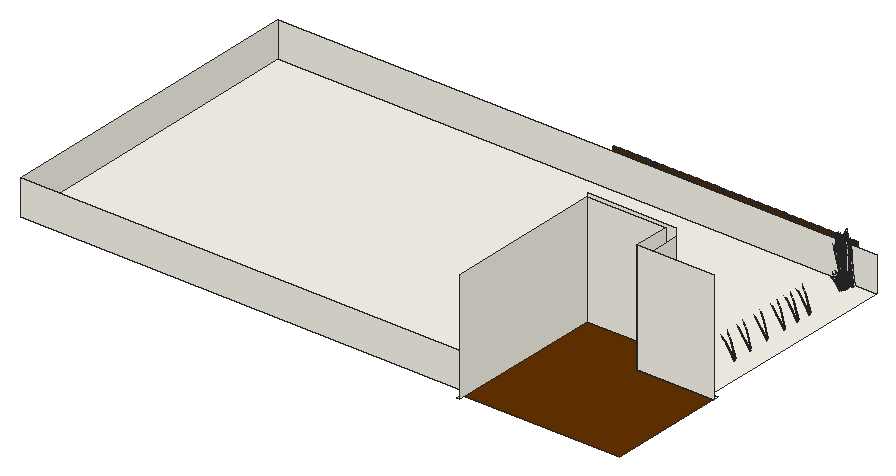
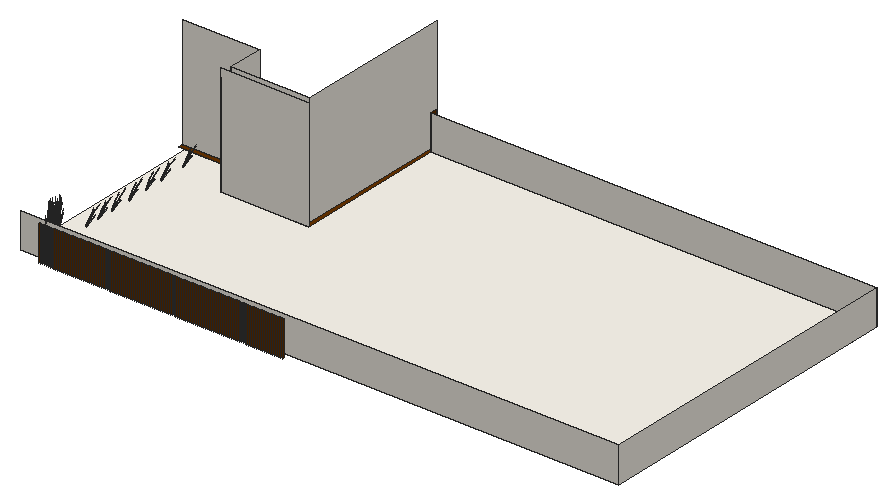
# SketchUp Ruby script. Lengths in inches.
U = 1.inch
M = Sketchup.active_model
def pt(a) = Geom::Point3d.new(a.map { |v| v * U })
def face(e, loops, mat)
  f = e.add_face(loops[0].map { |a| pt(a) })
  loops[1..].each { |l| e.add_face(l.map { |a| pt(a) }).erase! }
  f.material = f.back_material = mat if mat
  f
end
# faces: each face lists its corners as indices into pts; further lists are holes
def faces(e, pts, list, mat = nil) = list.each { |f| face(e, (f[0].is_a?(Array) ? f : [f]).map { |l| l.map { |i| pts[i] } }, mat) }
# xy, xz, yz: faces in a plane at the given z, y or x. An outline is a flat list of corners, or four numbers for a rectangle; further outlines are holes
def ring(l) = l.size == 4 ? [[l[0], l[1]], [l[2], l[1]], [l[2], l[3]], [l[0], l[3]]] : l.each_slice(2).to_a
def flat(e, list, mat, &to3) = list.each { |f| face(e, (f[0].is_a?(Array) ? f : [f]).map { |l| ring(l).map { |u, v| to3.(u, v) } }, mat) }
def xy(e, z, list, mat = nil) = flat(e, list, mat) { |x, y| [x, y, z] }
def xz(e, y, list, mat = nil) = flat(e, list, mat) { |x, z| [x, y, z] }
def yz(e, x, list, mat = nil) = flat(e, list, mat) { |y, z| [x, y, z] }
def lines(e, pts, list) = list.each { |a, b| e.add_line(pt(pts[a]), pt(pts[b])) }
# prism: a flat outline (further loops are holes) pulled along v
def prism(e, loops, v, mat = nil)
  f = face(e, loops, mat); d = Geom::Vector3d.new(v.map { |x| x * U })
  f.pushpull(f.normal.samedirection?(d) ? d.length : -d.length)
end
def box(e, o, s, mat = nil) = prism(e, [[o, [o[0] + s[0], o[1], o[2]], [o[0] + s[0], o[1] + s[1], o[2]], [o[0], o[1] + s[1], o[2]]]], [0, 0, s[2]], mat)
def at(x, y, z, deg = 0) = Geom::Transformation.translation(pt([x, y, z])) * Geom::Transformation.rotation(ORIGIN, Z_AXIS, deg.degrees)
def axes(o, x, y, z) = Geom::Transformation.new([*x, 0, *y, 0, *z, 0, *pt(o).to_a, 1])
def part(name) = M.definitions.add(name)
# library, detail: a bought-in or finely detailed component or shape, given as its bounding box
def library(name, o, s) = part(name).tap { |d| box(d.entities, o, s) }
def detail(e, o, s) = box(e.add_group.entities, o, s)
def put(e, d, t, mat = nil) = e.add_instance(d, t).tap { |i| i.material = mat if mat }
def group(e, t, mat = nil) = e.add_group.tap { |g| g.transformation = t; g.material = mat if mat }.entities
root = M.entities
M.materials.add("C01_Vanilla_Cream").color = [255, 251, 241]
M.materials.add("C08_Toffee_Ember").color = [102, 51, 0]
M.materials.add("LightPink_Translucent").color = [144, 107, 117]
M.materials["LightPink_Translucent"].alpha = 0.75
c1 = part("blade")
p = [[2.15,0.21,22],[0,0.17,0],[0.09,0.45,0],[2.18,0.31,22],[2.29,0.31,22],[0.38,0.45,0],
  [2.48,0.24,33],[2.49,0.24,33],[2.48,0.22,33]]
faces(c1.entities,p,[[0,1,2,3],[4,5,2,3],[6,3,4,7],[8,0,3,6]])
c2 = part("seeds")
p = [[0.3,-0.1,1.38],[-0.01,-0.03,1.59],[-0.01,-0.03,0.03],[0.14,-0.07,-0.07],[0.29,-0.03,3],[0.15,0.01,3.11]]
faces(c2.entities,p,[[0,1,2,3],[1,0,4,5]],"LightPink_Translucent")
c3 = part("blade with seeds")
put(c3.entities,c1,at(0,0,0))
put(c3.entities,c2,axes([2.4,0.25,30.99],[1.5799,-0.05474,1.17369],[-0.12525,1.92788,0.29478],[-0.07173,-0.02425,1.56792]))
xy(root,510,[[531,12,531,180,621.41,180,621.41,144,693.41,144,693.41,138,615.41,138,615.41,174,535,174,535,12],[75,24,531,24,531,180,621.41,180,621.41,144,687.41,144,687.41,354,75,354]],"C01_Vanilla_Cream")
xy(root,510,[[531,18,693.41,18,693.41,144,621.41,144,621.41,180,531,180]],"C08_Toffee_Ember")
xz(root,24,[[75,510,531,546]],"C01_Vanilla_Cream")
xz(root,138,[[615.41,510,693.41,624]],"C01_Vanilla_Cream")
xz(root,174,[[535,510,615.41,624]],"C01_Vanilla_Cream")
xz(root,180,[[531,510,621.41,624]],"C01_Vanilla_Cream")
xz(root,354,[[75,510,687.41,546]],"C01_Vanilla_Cream")
yz(root,75,[[24,510,354,546]],"C01_Vanilla_Cream")
yz(root,413.02,[[360,510,361.11,546]],"C08_Toffee_Ember")
yz(root,415.03,[[360,510,361.11,546]],"C08_Toffee_Ember")
yz(root,417.05,[[360,510,361.11,546]],"C08_Toffee_Ember")
yz(root,419.07,[[360,510,361.11,546]],"C08_Toffee_Ember")
yz(root,421.09,[[360,510,361.11,546]],"C08_Toffee_Ember")
yz(root,423.1,[[360,510,361.11,546]],"C08_Toffee_Ember")
yz(root,425.12,[[360,510,361.11,546]],"C08_Toffee_Ember")
yz(root,427.14,[[360,510,361.11,546]],"C08_Toffee_Ember")
yz(root,429.16,[[360,510,361.09,546]],"C08_Toffee_Ember")
yz(root,431.17,[[360,510,361.09,546]],"C08_Toffee_Ember")
yz(root,433.19,[[360,510,361.09,546]],"C08_Toffee_Ember")
yz(root,435.21,[[360,510,361.09,546]],"C08_Toffee_Ember")
yz(root,437.22,[[360,510,361.09,546]],"C08_Toffee_Ember")
yz(root,439.24,[[360,510,361.09,546]],"C08_Toffee_Ember")
yz(root,441.26,[[360,510,361.09,546]],"C08_Toffee_Ember")
yz(root,443.28,[[360,510,361.09,546]],"C08_Toffee_Ember")
yz(root,445.29,[[360,510,361.09,546]],"C08_Toffee_Ember")
yz(root,447.31,[[360,510,361.09,546]],"C08_Toffee_Ember")
yz(root,449.33,[[360,510,361.09,546]],"C08_Toffee_Ember")
yz(root,451.34,[[360,510,361.09,546]],"C08_Toffee_Ember")
yz(root,453.36,[[360,510,361.09,546]],"C08_Toffee_Ember")
yz(root,455.38,[[360,510,361.09,546]],"C08_Toffee_Ember")
yz(root,457.4,[[360,510,361.09,546]],"C08_Toffee_Ember")
yz(root,459.41,[[360,510,361.09,546]],"C08_Toffee_Ember")
yz(root,461.43,[[360,510,361.09,546]],"C08_Toffee_Ember")
yz(root,463.45,[[360,510,361.09,546]],"C08_Toffee_Ember")
yz(root,465.47,[[360,510,361.09,546]],"C08_Toffee_Ember")
yz(root,467.48,[[360,510,361.09,546]],"C08_Toffee_Ember")
yz(root,469.5,[[360,510,361.09,546]],"C08_Toffee_Ember")
yz(root,471.52,[[360,510,361.09,546]],"C08_Toffee_Ember")
yz(root,473.53,[[360,510,361.1875,546]],"C08_Toffee_Ember")
yz(root,475.55,[[360,510,361.1875,546]],"C08_Toffee_Ember")
yz(root,477.57,[[360,510,361.1875,546]],"C08_Toffee_Ember")
yz(root,479.59,[[360,510,361.1875,546]],"C08_Toffee_Ember")
yz(root,481.6,[[360,510,361.1875,546]],"C08_Toffee_Ember")
yz(root,483.62,[[360,510,361.1875,546]],"C08_Toffee_Ember")
yz(root,485.64,[[360,510,361.1875,546]],"C08_Toffee_Ember")
yz(root,487.66,[[360,510,361.1875,546]],"C08_Toffee_Ember")
yz(root,489.67,[[360,510,361.1875,546]],"C08_Toffee_Ember")
yz(root,491.69,[[360,510,361.1875,546]],"C08_Toffee_Ember")
yz(root,493.71,[[360,510,361.1875,546]],"C08_Toffee_Ember")
yz(root,495.72,[[360,510,361.1875,546]],"C08_Toffee_Ember")
yz(root,497.74,[[360,510,361.1875,546]],"C08_Toffee_Ember")
yz(root,499.76,[[360,510,361.1875,546]],"C08_Toffee_Ember")
yz(root,501.78,[[360,510,361.1875,546]],"C08_Toffee_Ember")
yz(root,503.79,[[360,510,361.1875,546]],"C08_Toffee_Ember")
yz(root,505.81,[[360,510,361.1875,546]],"C08_Toffee_Ember")
yz(root,507.83,[[360,510,361.1875,546]],"C08_Toffee_Ember")
yz(root,509.84,[[360,510,361.1875,546]],"C08_Toffee_Ember")
yz(root,511.86,[[360,510,361.1875,546]],"C08_Toffee_Ember")
yz(root,513.88,[[360,510,361.1875,546]],"C08_Toffee_Ember")
yz(root,515.9,[[360,510,361.1875,546]],"C08_Toffee_Ember")
yz(root,517.91,[[360,510,361.1875,546]],"C08_Toffee_Ember")
yz(root,519.93,[[360,510,361.1875,546]],"C08_Toffee_Ember")
yz(root,521.95,[[360,510,361.1875,546]],"C08_Toffee_Ember")
yz(root,523.97,[[360,510,361.1875,546]],"C08_Toffee_Ember")
yz(root,525.98,[[360,510,361.1875,546]],"C08_Toffee_Ember")
yz(root,528,[[360,510,361.1875,546]],"C08_Toffee_Ember")
yz(root,530.02,[[360,510,361.1875,546]],"C08_Toffee_Ember")
yz(root,531,[[18,510,24,546]],"C08_Toffee_Ember")
yz(root,532.03,[[360,510,361.1875,546]],"C08_Toffee_Ember")
yz(root,534.05,[[360,510,361.1875,546]],"C08_Toffee_Ember")
yz(root,535,[[12,510,174,624]],"C01_Vanilla_Cream")
yz(root,536.07,[[360,510,361.1875,546]],"C08_Toffee_Ember")
yz(root,538.09,[[360,510,361.1875,546]],"C08_Toffee_Ember")
yz(root,540.1,[[360,510,361.1875,546]],"C08_Toffee_Ember")
yz(root,542.12,[[360,510,361.1875,546]],"C08_Toffee_Ember")
yz(root,544.14,[[360,510,361.1875,546]],"C08_Toffee_Ember")
yz(root,546.15,[[360,510,361.1875,546]],"C08_Toffee_Ember")
yz(root,548.17,[[360,510,361.1875,546]],"C08_Toffee_Ember")
yz(root,550.1875,[[360,510,361.1875,546]],"C08_Toffee_Ember")
yz(root,552.21,[[360,510,361.1875,546]],"C08_Toffee_Ember")
yz(root,554.22,[[360,510,361.1875,546]],"C08_Toffee_Ember")
yz(root,556.24,[[360,510,361.1875,546]],"C08_Toffee_Ember")
yz(root,558.26,[[360,510,361.1875,546]],"C08_Toffee_Ember")
yz(root,560.28,[[360,510,361.1875,546]],"C08_Toffee_Ember")
yz(root,562.29,[[360,510,361.1875,546]],"C08_Toffee_Ember")
yz(root,564.31,[[360,510,361.1875,546]],"C08_Toffee_Ember")
yz(root,566.33,[[360,510,361.1875,546]],"C08_Toffee_Ember")
yz(root,568.34,[[360,510,361.1875,546]],"C08_Toffee_Ember")
yz(root,570.36,[[360,510,361.1875,546]],"C08_Toffee_Ember")
yz(root,572.38,[[360,510,361.1875,546]],"C08_Toffee_Ember")
yz(root,574.4,[[360,510,361.1875,546]],"C08_Toffee_Ember")
yz(root,576.41,[[360,510,361.1875,546]],"C08_Toffee_Ember")
yz(root,578.43,[[360,510,361.1875,546]],"C08_Toffee_Ember")
yz(root,580.45,[[360,510,361.1875,546]],"C08_Toffee_Ember")
yz(root,582.47,[[360,510,361.1875,546]],"C08_Toffee_Ember")
yz(root,584.48,[[360,510,361.1875,546]],"C08_Toffee_Ember")
yz(root,586.5,[[360,510,361.1875,546]],"C08_Toffee_Ember")
yz(root,588.52,[[360,510,361.1875,546]],"C08_Toffee_Ember")
yz(root,590.53,[[360,510,361.1875,546]],"C08_Toffee_Ember")
yz(root,592.55,[[360,510,361.1875,546]],"C08_Toffee_Ember")
yz(root,594.57,[[360,510,361.1875,546]],"C08_Toffee_Ember")
yz(root,596.59,[[360,510,361.1875,546]],"C08_Toffee_Ember")
yz(root,598.6,[[360,510,361.13,546]],"C08_Toffee_Ember")
yz(root,600.62,[[360,510,361.13,546]],"C08_Toffee_Ember")
yz(root,602.64,[[360,510,361.13,546]],"C08_Toffee_Ember")
yz(root,604.65,[[360,510,361.13,546]],"C08_Toffee_Ember")
yz(root,606.67,[[360,510,361.13,546]],"C08_Toffee_Ember")
yz(root,608.6875,[[360,510,361.13,546]],"C08_Toffee_Ember")
yz(root,610.71,[[360,510,361.13,546]],"C08_Toffee_Ember")
yz(root,612.72,[[360,510,361.13,546]],"C08_Toffee_Ember")
yz(root,614.74,[[360,510,361.13,546]],"C08_Toffee_Ember")
yz(root,615.41,[[138,510,174,624]],"C01_Vanilla_Cream")
yz(root,616.76,[[360,510,361.13,546]],"C08_Toffee_Ember")
yz(root,618.78,[[360,510,361.13,546]],"C08_Toffee_Ember")
yz(root,620.79,[[360,510,361.13,546]],"C08_Toffee_Ember")
yz(root,621.41,[[144,510,180,615]],"C01_Vanilla_Cream")
yz(root,622.81,[[360,510,361.13,546]],"C08_Toffee_Ember")
yz(root,624.83,[[360,510,361.13,546]],"C08_Toffee_Ember")
yz(root,626.84,[[360,510,361.13,546]],"C08_Toffee_Ember")
yz(root,628.86,[[360,510,361.13,546]],"C08_Toffee_Ember")
yz(root,630.88,[[360,510,361.13,546]],"C08_Toffee_Ember")
yz(root,632.9,[[360,510,361.13,546]],"C08_Toffee_Ember")
yz(root,634.91,[[360,510,361.13,546]],"C08_Toffee_Ember")
yz(root,636.93,[[360,510,361.13,546]],"C08_Toffee_Ember")
yz(root,638.95,[[360,510,361.13,546]],"C08_Toffee_Ember")
yz(root,640.97,[[360,510,361.13,546]],"C08_Toffee_Ember")
yz(root,642.98,[[360,510,361,546]],"C08_Toffee_Ember")
yz(root,645,[[360,510,361,546]],"C08_Toffee_Ember")
yz(root,647.02,[[360,510,361,546]],"C08_Toffee_Ember")
yz(root,649.03,[[360,510,361,546]],"C08_Toffee_Ember")
yz(root,651.05,[[360,510,361,546]],"C08_Toffee_Ember")
yz(root,653.07,[[360,510,361,546]],"C08_Toffee_Ember")
yz(root,655.09,[[360,510,361,546]],"C08_Toffee_Ember")
yz(root,657.1,[[360,510,361,546]],"C08_Toffee_Ember")
yz(root,659.12,[[360,510,361,546]],"C08_Toffee_Ember")
yz(root,661.14,[[360,510,361,546]],"C08_Toffee_Ember")
yz(root,663.15,[[360,510,361,546]],"C08_Toffee_Ember")
put(root,c3,axes([662.41,340.34,511.24],[0.0165,0.08998,1.46364],[-0.33262,0.46992,-0.2236],[-0.23626,-0.02369,0.24931]))
put(root,c3,axes([662.23,342.86,511.24],[0.08727,0.05704,1.46364],[0.14797,0.52853,-0.2236],[-0.19341,0.11271,0.24931]))
put(root,c3,axes([665.12,347.62,512.15],[0.12702,0.15896,1.18691],[-0.2927,0.4321,-0.25526],[-0.30054,-0.10328,0.50747]))
put(root,c3,axes([664.59,341.16,511.71],[-0.67676,-0.09361,-0.51753],[0.14281,-0.57742,-0.13583],[-0.20196,-0.06997,1.14236]))
put(root,c3,axes([664.67,348.68,511.24],[0.0165,0.08998,1.46364],[-0.33262,0.46992,-0.2236],[-0.23626,-0.02369,0.24931]))
put(root,c3,axes([663.7,342.25,511.67],[-0.60889,-0.28548,-0.4121],[0.36394,-0.51192,0],[-0.13868,-0.06502,1.30728]))
put(root,c3,axes([663.43,338,511.24],[-0.06302,0.07522,1.46364],[-0.63686,0.16217,-0.2236],[-0.15385,-0.14752,0.24931]))
put(root,c3,axes([664.07,342.59,511.97],[-0.40676,0.57214,0],[-0.68052,-0.31907,-0.42834],[-0.15499,-0.07267,1.3588]))
put(root,c3,axes([663.03,338.29,511.77],[-0.18768,0.46622,-0.03231],[-0.57763,-0.14342,-0.14649],[-0.0877,-0.07626,0.48318]))
put(root,c3,axes([664.49,351.2,511.24],[0.08727,0.05704,1.46364],[0.14797,0.52853,-0.2236],[-0.19341,0.11271,0.24931]))
put(root,c3,axes([665.35,341.24,512.21],[-0.65687,0.37907,-0.24149],[-0.43681,-0.53562,-0.41502],[-0.16207,-0.0544,1.32557]))
put(root,c3,axes([662.72,340.42,511.97],[-0.81352,0,0],[0,-0.63814,-0.42834],[0,-0.14534,1.3588]))
put(root,c3,axes([663.87,342.04,511.68],[-0.15283,-0.49751,-0.25712],[0.60696,-0.14127,0.25712],[-0.12236,-0.05737,1.15348]))
put(root,c3,axes([665.79,341.66,511.71],[-0.43821,0.42916,-0.51753],[-0.54436,-0.38915,-0.13583],[-0.1756,0.10706,1.14236]))
put(root,c3,axes([663.35,340.25,511.93],[-0.60515,0.48003,0.25528],[-0.60552,-0.47498,-0.30288],[-0.02113,-0.13632,1.36855]))
put(root,c3,axes([666.09,341.41,512.05],[-0.63528,-0.45956,-0.20909],[0.53456,-0.51604,0.45758],[-0.17107,0.05376,1.39619]))
put(root,c3,axes([664.9375,340.97,511.83],[-0.39083,-0.47924,-0.37133],[0.59199,-0.33747,0.17871],[-0.12647,-0.0593,1.19224]))
put(root,c3,axes([666.84,349.5,511.71],[-0.67676,-0.09361,-0.51753],[0.14281,-0.57742,-0.13583],[-0.20196,-0.06997,1.14236]))
put(root,c3,axes([665.77,341.32,511.83],[-0.70648,0.03525,-0.37133],[-0.06389,-0.58508,0.17871],[-0.12647,0.0593,1.19224]))
put(root,c3,axes([665.95,350.59,511.67],[-0.60889,-0.28548,-0.4121],[0.36394,-0.51192,0],[-0.13868,-0.06502,1.30728]))
put(root,c3,axes([665.6875,346.34,511.24],[-0.06302,0.07522,1.46364],[-0.63686,0.16217,-0.2236],[-0.15385,-0.14752,0.24931]))
put(root,c3,axes([666.33,350.94,511.97],[-0.40676,0.57214,0],[-0.68052,-0.31907,-0.42834],[-0.15499,-0.07267,1.3588]))
put(root,c3,axes([664.99,341.25,512.02],[0.17244,-0.67657,-0.19446],[0.81759,0.11793,0.42555],[-0.14286,-0.09343,1.29846]))
put(root,c3,axes([665.29,341.41,512.17],[-0.12551,0.50956,0.12018],[-0.6132,-0.08845,-0.34318],[-0.1116,-0.05232,1.05198]))
put(root,c3,axes([668.17,169.73,512.15],[0.2261,0.04687,1.18691],[0.14573,0.47875,-0.25526],[-0.30712,0.08962,0.50747]))
put(root,c3,axes([668.17,197.18,512.15],[0.2261,0.04687,1.18691],[0.14573,0.47875,-0.25526],[-0.30712,0.08962,0.50747]))
put(root,c3,axes([668.17,217.48,512.15],[0.2261,0.04687,1.18691],[0.14573,0.47875,-0.25526],[-0.30712,0.08962,0.50747]))
put(root,c3,axes([668.17,239.17,512.15],[0.2261,0.04687,1.18691],[0.14573,0.47875,-0.25526],[-0.30712,0.08962,0.50747]))
put(root,c3,axes([668.17,261.02,512.15],[0.2261,0.04687,1.18691],[0.14573,0.47875,-0.25526],[-0.30712,0.08962,0.50747]))
put(root,c3,axes([668.17,277.88,512.15],[0.2261,0.04687,1.18691],[0.14573,0.47875,-0.25526],[-0.30712,0.08962,0.50747]))
put(root,c3,axes([668.17,293.21,512.15],[0.2261,0.04687,1.18691],[0.14573,0.47875,-0.25526],[-0.30712,0.08962,0.50747]))
put(root,c3,axes([666.51,342.83,511.67],[-0.60889,0.28548,-0.4121],[-0.36394,-0.51192,0],[-0.13868,0.06502,1.30728]))
put(root,c3,axes([662.91,339.98,511.67],[0,-0.57097,-0.4121],[0.72788,0,0],[0,-0.13004,1.30728]))
put(root,c3,axes([666.55,342.67,511.82],[-0.40169,-0.57414,-0.04268],[0.68052,-0.31907,0.42834],[-0.16769,0.05466,1.35813]))
put(root,c3,axes([665.58,351.76,512.15],[0.2053,-0.09007,1.18691],[0.50689,0.27159,-0.25526],[-0.15087,0.235,0.50747]))
put(root,c3,axes([666.37,342.6,511.68],[-0.60696,-0.14127,-0.25712],[0.15283,-0.49751,0.25712],[-0.12236,0.05737,1.15348]))
put(root,c3,axes([665.29,346.63,511.77],[-0.18768,0.46622,-0.03231],[-0.57763,-0.14342,-0.14649],[-0.0877,-0.07626,0.48318]))
put(root,c3,axes([664.81,340.64,512.21],[-0.73268,-0.27244,-0.24149],[0.35279,-0.57501,-0.41502],[-0.02303,-0.14118,1.32557]))
put(root,c3,axes([666.15,346.04,512.15],[-0.0394,0.18678,1.18691],[-0.57594,0.15636,-0.25526],[-0.13463,-0.24142,0.50747]))
put(root,c3,axes([667.61,349.58,512.21],[-0.65687,0.37907,-0.24149],[-0.43681,-0.53562,-0.41502],[-0.16207,-0.0544,1.32557]))
put(root,c3,axes([663.47,342.99,512.34],[0.59102,-0.10111,0.05401],[0.13587,0.40735,-0.71633],[-0.03747,0.2062,0.64209]))
put(root,c3,axes([666.26,341.16,512.21],[0.07581,0.65151,-0.24149],[-0.7896,0.03939,-0.41502],[-0.13904,0.08678,1.32557]))
put(root,c3,axes([664.48,340.0625,511.74],[-0.26718,-0.5855,-0.57963],[0.76964,-0.21087,-0.15213],[-0.02953,-0.19827,1.27944]))
put(root,c3,axes([669.04,167.41,512.15],[0.12702,0.15896,1.18691],[-0.2927,0.4321,-0.25526],[-0.30054,-0.10328,0.50747]))
put(root,c3,axes([669.04,194.87,512.15],[0.12702,0.15896,1.18691],[-0.2927,0.4321,-0.25526],[-0.30054,-0.10328,0.50747]))
put(root,c3,axes([669.04,236.86,512.15],[0.12702,0.15896,1.18691],[-0.2927,0.4321,-0.25526],[-0.30054,-0.10328,0.50747]))
put(root,c3,axes([669.04,258.7,512.15],[0.12702,0.15896,1.18691],[-0.2927,0.4321,-0.25526],[-0.30054,-0.10328,0.50747]))
put(root,c3,axes([669.04,290.9,512.15],[0.12702,0.15896,1.18691],[-0.2927,0.4321,-0.25526],[-0.30054,-0.10328,0.50747]))
put(root,c3,axes([669.04,215.16,512.15],[0.12702,0.15896,1.18691],[-0.2927,0.4321,-0.25526],[-0.30054,-0.10328,0.50747]))
put(root,c3,axes([669.04,275.5625,512.15],[0.12702,0.15896,1.18691],[-0.2927,0.4321,-0.25526],[-0.30054,-0.10328,0.50747]))
put(root,c3,axes([664.98,348.76,511.97],[-0.81352,0,0],[0,-0.63814,-0.42834],[0,-0.14534,1.3588]))
put(root,c3,axes([666.125,350.38,511.68],[-0.15283,-0.49751,-0.25712],[0.60696,-0.14127,0.25712],[-0.12236,-0.05737,1.15348]))
put(root,c3,axes([663.22,339.99,511.68],[0.45414,-0.35624,-0.25712],[0.45414,0.35624,0.25712],[0,-0.11474,1.15348]))
put(root,c3,axes([665.27,337.69,511.77],[-0.44958,0.32756,-0.03231],[-0.41194,-0.35875,-0.14649],[-0.029,-0.10165,0.48318]))
put(root,c3,axes([665.09,340.92,511.96],[0.82229,0.1203,0.37976],[-0.16734,0.67942,0.14902],[-0.12017,-0.06561,1.31851]))
put(root,c3,axes([668.05,350,511.71],[-0.43821,0.42916,-0.51753],[-0.54436,-0.38915,-0.13583],[-0.1756,0.10706,1.14236]))
put(root,c3,axes([665.61,348.59,511.93],[-0.60515,0.48003,0.25528],[-0.60552,-0.47498,-0.30288],[-0.02113,-0.13632,1.36855]))
put(root,c3,axes([668.59,168.48,511.24],[0.0165,0.08998,1.46364],[-0.33262,0.46992,-0.2236],[-0.23626,-0.02369,0.24931]))
put(root,c3,axes([668.59,195.93,511.24],[0.0165,0.08998,1.46364],[-0.33262,0.46992,-0.2236],[-0.23626,-0.02369,0.24931]))
put(root,c3,axes([668.59,237.92,511.24],[0.0165,0.08998,1.46364],[-0.33262,0.46992,-0.2236],[-0.23626,-0.02369,0.24931]))
put(root,c3,axes([668.59,259.77,511.24],[0.0165,0.08998,1.46364],[-0.33262,0.46992,-0.2236],[-0.23626,-0.02369,0.24931]))
put(root,c3,axes([668.59,291.96,511.24],[0.0165,0.08998,1.46364],[-0.33262,0.46992,-0.2236],[-0.23626,-0.02369,0.24931]))
put(root,c3,axes([668.59,216.23,511.24],[0.0165,0.08998,1.46364],[-0.33262,0.46992,-0.2236],[-0.23626,-0.02369,0.24931]))
put(root,c3,axes([668.59,276.63,511.24],[0.0165,0.08998,1.46364],[-0.33262,0.46992,-0.2236],[-0.23626,-0.02369,0.24931]))
put(root,c3,axes([668.35,349.76,512.05],[-0.63528,-0.45956,-0.20909],[0.53456,-0.51604,0.45758],[-0.17107,0.05376,1.39619]))
put(root,c3,axes([667.19,349.3125,511.83],[-0.39083,-0.47924,-0.37133],[0.59199,-0.33747,0.17871],[-0.12647,-0.0593,1.19224]))
put(root,c3,axes([665.55,342.1,511.82],[-0.65588,-0.25634,0],[0.31565,-0.53263,0],[0,0,1.35047]))
put(root,c3,axes([667.0625,342.74,511.97],[0.40676,0.57214,0],[-0.68052,0.31907,-0.42834],[-0.15499,0.07267,1.3588]))
